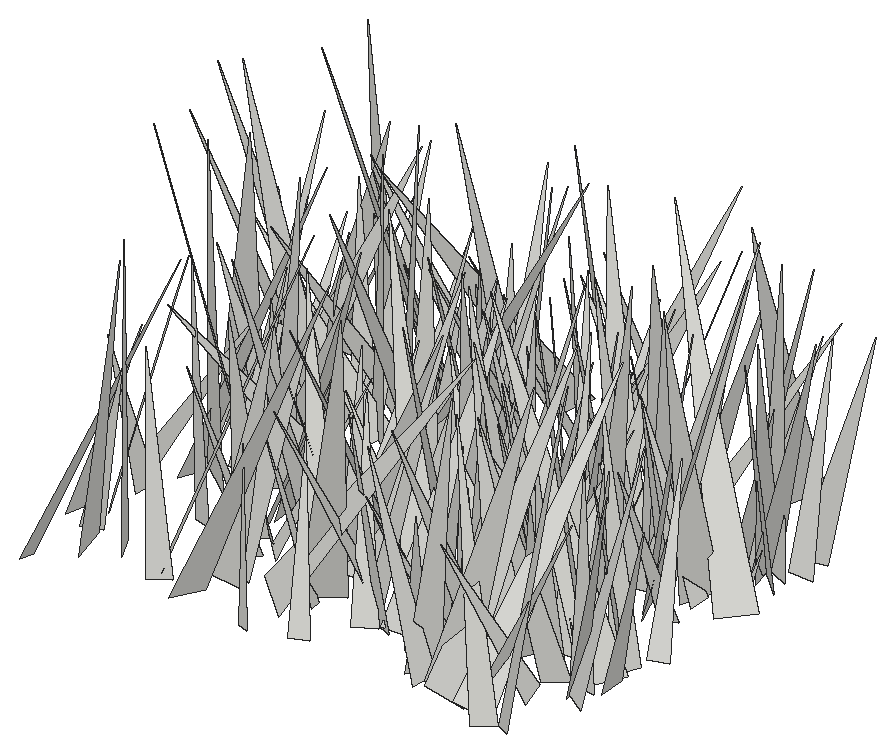
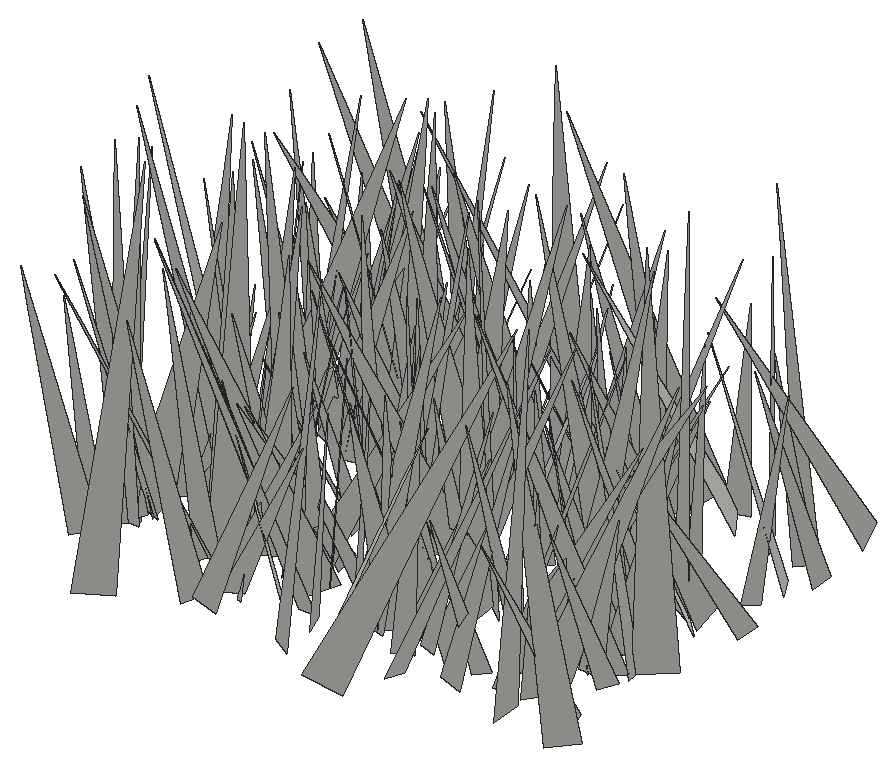
# SketchUp Ruby script. Lengths in inches.
U = 1.inch
M = Sketchup.active_model
def pt(a) = Geom::Point3d.new(a.map { |v| v * U })
def face(e, loops, mat)
  f = e.add_face(loops[0].map { |a| pt(a) })
  loops[1..].each { |l| e.add_face(l.map { |a| pt(a) }).erase! }
  f.material = f.back_material = mat if mat
  f
end
# faces: each face lists its corners as indices into pts; further lists are holes
def faces(e, pts, list, mat = nil) = list.each { |f| face(e, (f[0].is_a?(Array) ? f : [f]).map { |l| l.map { |i| pts[i] } }, mat) }
# xy, xz, yz: faces in a plane at the given z, y or x. An outline is a flat list of corners, or four numbers for a rectangle; further outlines are holes
def ring(l) = l.size == 4 ? [[l[0], l[1]], [l[2], l[1]], [l[2], l[3]], [l[0], l[3]]] : l.each_slice(2).to_a
def flat(e, list, mat, &to3) = list.each { |f| face(e, (f[0].is_a?(Array) ? f : [f]).map { |l| ring(l).map { |u, v| to3.(u, v) } }, mat) }
def xy(e, z, list, mat = nil) = flat(e, list, mat) { |x, y| [x, y, z] }
def xz(e, y, list, mat = nil) = flat(e, list, mat) { |x, z| [x, y, z] }
def yz(e, x, list, mat = nil) = flat(e, list, mat) { |y, z| [x, y, z] }
def lines(e, pts, list) = list.each { |a, b| e.add_line(pt(pts[a]), pt(pts[b])) }
# prism: a flat outline (further loops are holes) pulled along v
def prism(e, loops, v, mat = nil)
  f = face(e, loops, mat); d = Geom::Vector3d.new(v.map { |x| x * U })
  f.pushpull(f.normal.samedirection?(d) ? d.length : -d.length)
end
def box(e, o, s, mat = nil) = prism(e, [[o, [o[0] + s[0], o[1], o[2]], [o[0] + s[0], o[1] + s[1], o[2]], [o[0], o[1] + s[1], o[2]]]], [0, 0, s[2]], mat)
def at(x, y, z, deg = 0) = Geom::Transformation.translation(pt([x, y, z])) * Geom::Transformation.rotation(ORIGIN, Z_AXIS, deg.degrees)
def axes(o, x, y, z) = Geom::Transformation.new([*x, 0, *y, 0, *z, 0, *pt(o).to_a, 1])
def part(name) = M.definitions.add(name)
# library, detail: a bought-in or finely detailed component or shape, given as its bounding box
def library(name, o, s) = part(name).tap { |d| box(d.entities, o, s) }
def detail(e, o, s) = box(e.add_group.entities, o, s)
def put(e, d, t, mat = nil) = e.add_instance(d, t).tap { |i| i.material = mat if mat }
def group(e, t, mat = nil) = e.add_group.tap { |g| g.transformation = t; g.material = mat if mat }.entities
root = M.entities
c1 = part("fur_instance\#9")
p = [[0.8125,0,1.79],[0.67,-0.02,1.48],[0,-0.11,0],[0,0.11,0]]
faces(c1.entities,p,[[0,1,2,3]])
put(root,c1,axes([138.46,445.25,-27.1],[-0.67807,6.71445,3.30984],[6.96597,-0.65101,2.74773],[-2.74118,-3.31527,6.16389]))
put(root,c1,axes([137.26,444.68,-27.1],[-1.4583,4.1794,0.64732],[4.14586,1.27741,1.09233],[-0.83566,-0.95598,4.28962]))
put(root,c1,axes([135.875,436.88,-27.1],[-3.46561,0.71078,2.1355],[1.4755,3.67824,1.17025],[1.69955,-1.74395,3.33859]))
put(root,c1,axes([134.85,433.95,-27.1],[4.46137,-0.22154,0.62784],[-0.29219,-4.4737,0.49769],[-0.59824,0.53291,4.43905]))
put(root,c1,axes([134.64,438.63,-27.1],[3.53802,-1.77872,0.68161],[-1.86523,-2.94336,2.00089],[0.38644,2.07817,3.41729]))
put(root,c1,axes([136.17,445.02,-27.1],[-2.24412,3.20659,0.81725],[3.00578,2.38826,-1.11699],[1.38398,0.01256,3.75108]))
put(root,c1,axes([135.39,447.88,-27.1],[4.11341,0.99659,0.14821],[0.94897,-4.04143,0.83763],[-0.33855,0.78037,4.1487]))
put(root,c1,axes([135.64,435.11,-27.1],[4.69542,3.0157,0.91715],[3.05189,-4.76105,0.03053],[-0.78841,-0.46959,5.58037]))
put(root,c1,axes([137.41,442.85,-27.1],[2.70621,-3.86796,1.26709],[-3.69816,-2.97221,-1.17466],[-1.70008,0.30833,4.57219]))
put(root,c1,axes([134.6875,449.55,-27.1],[2.49015,-6.48815,0.76577],[-6.33726,-2.19962,1.97082],[1.58797,1.39602,6.66429]))
put(root,c1,axes([135.39,443.14,-27.1],[5.72891,-5.77899,0.7373],[-5.79412,-5.75966,-0.12335],[-0.60698,0.43635,8.13646]))
put(root,c1,axes([135.65,430.11,-27.1],[6.20269,2.14266,0.41588],[1.88774,-5.89525,2.21806],[-1.09562,1.97291,6.17613]))
put(root,c1,axes([136.48,439.63,-27.1],[3.1839,3.43631,0.24845],[3.39454,-3.18669,0.57383],[-0.5891,0.20968,4.64932]))
put(root,c1,axes([136.17,433.32,-27.1],[2.52401,-3.24586,0.70539],[-3.32076,-2.44552,0.62916],[0.07602,0.94215,4.0633]))
put(root,c1,axes([141.53,442.02,-27.1],[-3.36679,-6.63148,1.92496],[-6.20382,1.96447,-4.08298],[-3.03226,3.34389,6.21619]))
put(root,c1,axes([137.76,447.41,-27.1],[3.42061,-2.16163,2.16053],[-2.46149,-3.8706,0.02453],[-1.81151,1.17767,4.04631]))
put(root,c1,axes([135.87,443.82,-27.1],[5.69454,1.71793,1.14191],[1.95584,-5.5622,-1.38552],[-0.6557,-1.67144,5.78441]))
put(root,c1,axes([137.82,440.1,-27.1],[1.84381,6.83005,0.32521],[6.75707,-1.87158,0.99709],[-1.04756,-0.05069,7.00393]))
put(root,c1,axes([139.02,443.38,-27.1],[-7.80525,1.8691,2.4402],[2.24771,8.01322,1.05174],[2.09664,-1.63243,7.95672]))
put(root,c1,axes([137.82,449,-27.1],[-7.27615,-1.41209,3.18772],[-1.2687,7.94356,0.62294],[3.24745,-0.06052,7.38568]))
put(root,c1,axes([138.12,432.84,-27.1],[5.01686,3.02729,2.73746],[3.17963,-5.61852,0.38618],[-2.55892,-1.04628,5.84673]))
put(root,c1,axes([137.42,439.07,-27.1],[-3.84702,-6.56229,2.86732],[-6.71624,4.43571,1.14075],[2.48541,1.82909,7.52076]))
put(root,c1,axes([136.5,438.68,-27.1],[6.82155,0.82248,0.97272],[0.53436,-6.65794,1.88216],[-1.15634,1.77527,6.60814]))
put(root,c1,axes([140.33,445.28,-27.1],[-4.08347,2.98679,1.40676],[3.27171,3.36098,2.36101],[-0.44252,-2.71247,4.47451]))
put(root,c1,axes([136.89,432.24,-27.1],[6.91292,1.02767,1.79019],[1.3308,-7.00178,-1.11957],[-1.57792,-1.40299,6.89863]))
put(root,c1,axes([139.17,436.13,-27.1],[1.89742,4.59885,2.05217],[4.78177,-2.33318,0.8074],[-1.57969,-1.53878,4.90894]))
put(root,c1,axes([137.47,444.66,-27.1],[3.73633,3.15118,1.53756],[3.50493,-3.41917,-1.50964],[-0.09758,-2.15258,4.64878]))
put(root,c1,axes([142.22,436.53,-27.1],[-6.33694,-5.31771,1.42218],[-5.44687,5.74429,-2.79146],[-0.79519,3.03026,7.78734]))
put(root,c1,axes([140.46,442.15,-27.1],[-5.57045,-1.42182,0.3414],[-1.0257,4.7578,3.07884],[1.04215,-2.91715,4.85512]))
put(root,c1,axes([139.31,447.74,-27.1],[-5.60645,-3.595,0.79099],[-2.74257,5.04084,3.47133],[2.4552,-2.57833,5.68385]))
put(root,c1,axes([138.93,441.08,-27.1],[6.1687,-0.67373,2.21616],[-0.70194,-6.55164,-0.0379],[-2.20738,0.2006,6.20527]))
put(root,c1,axes([139,446.24,-27.1],[0.94432,5.62245,1.27282],[5.76049,-0.87093,-0.42662],[0.22085,-1.32412,5.68522]))
put(root,c1,axes([136.49,444.21,-27.1],[1.93796,6.92662,2.2466],[6.80944,-0.90011,-3.09877],[2.58009,-2.82714,6.49087]))
put(root,c1,axes([142.74,446.75,-27.1],[-5.1387,-6.17044,1.38685],[-6.22365,4.61615,-2.52214],[-1.12419,2.64967,7.62361]))
put(root,c1,axes([137.97,442.4,-27.1],[3.87779,-2.1954,0.31482],[-2.2129,-3.78759,0.8446],[0.14815,0.88911,4.37535]))
put(root,c1,axes([140.57,431.82,-27.1],[1.59272,-3.9303,2.28796],[-4.37909,-1.9795,-0.352],[-1.22702,1.96293,4.22612]))
put(root,c1,axes([140.82,448.55,-27.1],[-1.81224,-5.34948,0.90018],[-5.42401,1.80193,-0.21131],[0.08596,0.92064,5.64415]))
put(root,c1,axes([139.6,437.65,-27.1],[2.64561,4.33348,1.24236],[4.47199,-2.70465,-0.08904],[-0.56902,-1.10798,5.07645]))
put(root,c1,axes([139.79,439.99,-27.1],[3.06125,-3.87557,0.82155],[-3.90702,-3.12527,-0.1848],[-0.65588,0.52812,4.93529]))
put(root,c1,axes([142.3,435.47,-27.1],[-1.49858,-3.44059,1.04989],[-3.40031,0.98374,-1.62968],[-1.17382,1.54281,3.38047]))
put(root,c1,axes([140.17,445.26,-27.1],[-3.26006,-5.04679,2.60885],[-5.29814,3.78652,0.70434],[2.05082,1.75965,5.96674]))
put(root,c1,axes([140.4,447.2,-27.1],[-1.29453,3.3269,0.92168],[3.25121,1.50588,-0.8692],[1.16077,-0.50757,3.46245]))
put(root,c1,axes([142.85,449.34,-27.1],[-6.28485,-0.79991,0.77187],[-0.56549,6.11624,1.73401],[0.95701,-1.63912,6.09364]))
put(root,c1,axes([140.27,432.24,-27.1],[5.9455,4.2001,0.21568],[4.05072,-5.81939,1.66213],[-1.13095,1.23699,7.08711]))
put(root,c1,axes([141.33,436.36,-27.1],[3.50702,-4.68842,0.88051],[-4.69288,-3.58696,-0.4079],[-0.85643,0.45629,5.84073]))
put(root,c1,axes([141.22,437.29,-27.1],[3.86213,1.08614,0.2172],[1.09096,-3.86634,-0.0646],[-0.19154,-0.12107,4.01143]))
put(root,c1,axes([143.96,437.25,-27.1],[-0.89834,-6.55906,1.37521],[-6.65422,0.70817,-0.96916],[-0.7961,1.48213,6.54897]))
put(root,c1,axes([143.14,447.02,-27.1],[-1.82356,-4.42835,0.39133],[-4.41286,1.85435,0.42054],[0.53859,0.19978,4.77062]))
put(root,c1,axes([144.49,451.57,-27.1],[4.16443,-6.48584,0.7003],[-5.50995,-3.94185,-3.74183],[-3.49241,-1.51483,6.7385]))
put(root,c1,axes([144.28,446.5,-27.1],[-0.56318,-3.80765,0.20803],[-3.75255,0.51599,-0.71463],[-0.67806,0.30692,3.78215]))
put(root,c1,axes([141.12,438.875,-27.1],[7.51831,-0.309,0.51299],[-0.23256,-7.46002,-1.08516],[-0.55186,-1.06592,7.446]))
put(root,c1,axes([143.74,439.35,-27.1],[-2.47,2.58512,1.49197],[2.74392,2.72878,-0.18549],[1.17462,-0.93843,3.57063]))
put(root,c1,axes([143,443.21,-27.1],[-4.52397,-6.09316,3.51067],[-6.34353,5.33763,1.08955],[3.03497,2.07386,7.51038]))
put(root,c1,axes([144.87,440.02,-27.1],[-3.28468,-3.33783,0.1825],[-3.30088,3.27904,0.56182],[0.52783,-0.26523,4.64915]))
put(root,c1,axes([142.43,433.98,-27.1],[0.67083,5.9533,2.27987],[6.17356,-0.03505,-1.72498],[1.58958,-2.37626,5.73727]))
put(root,c1,axes([142.48,433.25,-27.1],[1.87666,-6.19619,1.68038],[-6.32701,-1.4881,1.57887],[1.08876,2.03251,6.27868]))
put(root,c1,axes([142.64,436.03,-27.1],[3.00056,3.161,0.00616],[3.13284,-2.97269,-0.58633],[0.42105,-0.40809,4.31874]))
put(root,c1,axes([144.56,443.53,-27.1],[-0.28609,-7.90952,0.17476],[-7.91116,0.28452,-0.07401],[-0.06767,0.17732,7.91434]))
put(root,c1,axes([144.39,438.13,-27.1],[-3.15103,-4.03715,0.66571],[-3.75697,3.18756,1.54769],[1.62077,-0.46003,4.88182]))
put(root,c1,axes([146.35,433.85,-27.1],[-3.92472,-1.58946,0.29836],[-1.61245,3.78584,-1.04222],[-0.12416,1.07696,4.10409]))
put(root,c1,axes([143.62,447.89,-27.1],[0.2783,-5.0487,0.14304],[-4.93686,-0.24166,1.07529],[1.0664,0.19877,4.94071]))
put(root,c1,axes([144.15,443.14,-27.1],[3.92282,-1.4058,1.44453],[-1.66907,-4.03753,0.60333],[-1.1301,1.0833,4.1232]))
put(root,c1,axes([146.07,447.01,-27.1],[-0.62718,-6.98929,2.39617],[-7.29856,0.2117,-1.29283],[-1.15016,2.46782,6.89725]))
put(root,c1,axes([145.92,434.93,-27.1],[2.97491,-4.25566,3.74848],[-5.0806,-3.88069,-0.37363],[-2.51977,2.80026,5.17891]))
put(root,c1,axes([145.31,430.88,-27.1],[1.49909,3.09185,1.25062],[3.12666,-1.78006,0.6529],[-1.16087,-0.8017,3.3735]))
put(root,c1,axes([145.91,449.82,-27.1],[-3.80651,-3.12707,0.03174],[-3.06593,3.74155,0.93273],[0.61617,-0.70095,4.83716]))
put(root,c1,axes([142.07,431.61,-27.1],[7.97011,-1.5942,0.50435],[-1.65185,-7.88792,1.1707],[-0.25934,1.24806,8.04323]))
put(root,c1,axes([145.84,445.64,-27.1],[-5.09281,3.29268,0.78292],[3.01884,5.05892,-1.63872],[1.53013,0.9783,5.83893]))
put(root,c1,axes([144.82,442.04,-27.1],[-1.49682,6.02983,3.22428],[6.74332,1.8484,-0.32627],[1.1325,-3.03643,6.20426]))
put(root,c1,axes([145.1,446.67,-27.1],[-2.61332,3.50076,2.27341],[3.90248,3.00092,-0.13507],[1.48133,-1.72983,4.36652]))
put(root,c1,axes([145.95,443.05,-27.1],[0.78964,4.34465,0.57519],[4.335,-0.86018,0.54605],[-0.64386,-0.46311,4.38193]))
put(root,c1,axes([146.01,441.5,-27.1],[2.63979,2.66437,0.28601],[2.37928,-2.51517,1.47039],[-1.23275,0.85099,3.4504]))
put(root,c1,axes([147.05,445.27,-27.1],[0.66208,3.60921,1.19442],[3.54519,-1.02396,1.12897],[-1.37285,-0.90361,3.49144]))
put(root,c1,axes([145.29,446.49,-27.1],[4.67947,-2.49587,0.44393],[-2.29207,-4.56374,-1.49753],[-1.08298,-1.12554,5.08765]))
put(root,c1,axes([143.25,443.24,-27.1],[7.82793,-0.68601,0.13891],[-0.69946,-7.6099,1.83483],[0.02566,1.8399,7.64072]))
put(root,c1,axes([145.86,436.43,-27.1],[-1.59343,4.55905,1.08338],[4.45907,1.82697,-1.12985],[1.44061,-0.61229,4.69546]))
put(root,c1,axes([145.58,444.2,-27.1],[5.69502,0.05498,1.49404],[0.36012,-5.7612,-1.16071],[-1.45103,-1.21405,5.57575]))
put(root,c1,axes([147.49,441.54,-27.1],[-3.18847,2.06393,0.29466],[1.98964,3.17316,-0.69666],[0.62286,0.42918,3.73374]))
put(root,c1,axes([146.5,442.32,-27.1],[4.01654,5.38759,0.39242],[5.219,-3.99648,1.45013],[-1.3936,0.56102,6.56169]))
put(root,c1,axes([148.5,437.5,-27.1],[-3.99734,1.08155,0.32432],[1.12476,3.91891,0.79421],[0.09918,-0.85212,4.0642]))
put(root,c1,axes([147.4375,431.52,-27.1],[-1.47,3.64091,0.87512],[3.73843,1.4809,0.11844],[0.21496,-0.85654,3.92467]))
put(root,c1,axes([147.6,448.16,-27.1],[-4.30965,-1.39305,1.63599],[-1.58025,4.5392,-0.29767],[1.45598,0.80324,4.51941]))
put(root,c1,axes([146.3125,445.99,-27.1],[-4.08433,-4.26667,3.28401],[-4.58243,4.91876,0.69141],[2.82675,1.80893,5.86585]))
put(root,c1,axes([149.05,437.01,-27.1],[2.27452,-5.56414,4.58515],[-6.58849,-3.55674,-1.04785],[-2.92831,3.68058,5.91904]))
put(root,c1,axes([147.09,443.36,-27.1],[-3.51133,-6.12863,1.17286],[-5.90116,3.69891,1.66117],[2.0278,0.152,6.86513]))
put(root,c1,axes([148.38,437.23,-27.1],[-2.55623,-6.61752,0.06611],[-6.61278,2.55692,0.25211],[0.25899,-0.02922,7.08959]))
put(root,c1,axes([147.51,450.23,-27.1],[-4.05006,-5.82532,2.03849],[-5.82326,4.4146,1.04584],[2.04438,1.03428,7.01738]))
put(root,c1,axes([148.43,435.33,-27.1],[-4.62318,-3.47557,0.41553],[-3.19467,4.47097,1.85217],[1.4305,-1.24775,5.47931]))
put(root,c1,axes([147.75,445.39,-27.1],[-1.86728,-3.21645,1.13397],[-3.16749,2.11482,0.78275],[1.26429,0.54787,3.63587]))
put(root,c1,axes([146.36,436.55,-27.1],[0.74046,6.81709,2.01452],[6.9144,-0.22063,-1.79488],[1.64984,-2.13492,6.61811]))
put(root,c1,axes([150.45,444.42,-27.1],[-1.24481,-6.10899,0.55091],[-5.80958,0.99391,-2.10566],[-1.96776,0.93016,5.86818]))
put(root,c1,axes([146.16,434.57,-27.1],[5.23004,-6.31048,0.45418],[-6.32662,-5.22094,0.31214],[-0.04891,0.54893,8.19012]))
put(root,c1,axes([148.82,433.72,-27.1],[-2.21571,3.96483,0.99922],[4.07213,2.24229,0.13245],[0.36886,-0.93805,4.54001]))
put(root,c1,axes([145.53,436.58,-27.1],[5.33015,-4.46349,0.382],[-4.4244,-5.15196,1.5366],[0.7024,1.41905,6.78027]))
put(root,c1,axes([148.25,434.95,-27.1],[3.95249,6.61953,0.92655],[6.54498,-4.05132,1.02412],[-1.35642,-0.25967,7.64143]))
put(root,c1,axes([149.41,434.05,-27.1],[1.51862,3.68557,2.40948],[4.21899,-1.94756,0.31991],[-1.2606,-2.07817,3.97332]))
put(root,c1,axes([149.16,445.26,-27.1],[-3.54566,-2.66431,1.6705],[-2.78653,3.82874,0.19209],[1.45754,0.83849,4.43096]))
put(root,c1,axes([149.42,439.99,-27.1],[-4.67336,-1.61213,2.14084],[-2.03116,4.93814,-0.71533],[1.7483,1.42769,4.89159]))
put(root,c1,axes([147.56,438.25,-27.1],[3.87683,-5.48097,2.21285],[-5.90731,-3.50163,1.67625],[0.20355,2.76859,6.50085]))
put(root,c1,axes([144.63,433.45,-27.1],[4.68753,6.76488,0.69054],[6.04009,-3.75687,-4.19721],[3.12373,-2.88717,7.07954]))
put(root,c1,axes([151.45,448.19,-27.1],[-3.62089,2.64212,0.01483],[2.58278,3.53416,0.96476],[-0.55698,-0.78788,4.37731]))
put(root,c1,axes([150.62,444.22,-27.1],[-4.55116,2.07867,0.64916],[1.93391,4.54938,-1.00919],[1.00113,0.66152,4.90056]))
put(root,c1,axes([148.16,444.66,-27.1],[1.07989,-3.22676,1.49499],[-3.22529,-0.23045,1.83235],[1.49815,1.82977,2.86716]))
put(root,c1,axes([152,447.87,-27.1],[-4.37284,2.10544,0.41102],[2.13916,4.20984,1.19366],[-0.16073,-1.25217,4.70423]))
put(root,c1,axes([151.1,445.63,-27.1],[-4.28874,-2.62611,1.19653],[-2.76089,4.3576,-0.33198],[0.84,0.91449,5.01792]))
put(root,c1,axes([149.01,441.76,-27.1],[-2.72966,-3.54913,3.67888],[-4.47058,3.67982,0.23296],[2.47878,2.72838,4.47136]))
put(root,c1,axes([151.71,449.55,-27.1],[-0.61117,-4.98438,1.28841],[-4.9544,0.21679,-1.51148],[-1.3993,1.40945,4.78884]))
put(root,c1,axes([152.01,437.91,-27.1],[-4.80614,1.67739,0.07303],[1.63862,4.73444,-0.90443],[0.36591,0.83033,5.00945]))
put(root,c1,axes([152.04,436.93,-27.1],[-4.34264,3.05124,0.46122],[3.07623,4.34339,0.23041],[0.24406,-0.45414,5.3024]))
put(root,c1,axes([148.8,448.32,-27.1],[3.81482,2.67004,0.71919],[2.75746,-3.58156,-1.32965],[0.20681,-1.49748,4.4625]))
put(root,c1,axes([149.95,438.84,-27.1],[-0.40221,-7.56998,1.93164],[-7.73436,0.65878,0.97125],[1.10251,1.85984,7.51818]))
put(root,c1,axes([149.92,437.72,-27.1],[-3.16207,-7.07316,1.24758],[-6.76016,3.39142,2.09364],[2.42619,0.2311,7.45956]))
put(root,c1,axes([149.51,443.8,-27.1],[3.96425,-0.56902,0.64503],[-0.79665,-3.57598,1.74151],[-0.32433,1.82859,3.60641]))
put(root,c1,axes([151.75,435.0625,-27.1],[-3.32799,-2.15223,0.18164],[-2.02775,3.22824,1.09879],[0.74386,-0.82886,3.80792]))
put(root,c1,axes([150.16,434.19,-27.1],[-2.57926,6.41675,1.59968],[6.21683,2.93816,-1.76197],[2.25493,-0.76079,6.68751]))
put(root,c1,axes([152.11,445.125,-27.1],[-4.3858,5.26104,2.02142],[5.54364,4.48874,0.34523],[1.01623,-1.78118,6.84066]))
put(root,c1,axes([150.25,441.11,-27.1],[0.10364,-5.95888,1.80759],[-6.13378,0.21397,1.05707],[1.07352,1.79787,5.86529]))
put(root,c1,axes([150.87,441.42,-27.1],[4.041,0.55824,1.1889],[0.26805,-4.11576,1.02147],[-1.28579,0.89645,3.94942]))
put(root,c1,axes([151.73,443.16,-27.1],[-3.94545,3.07895,0.18102],[2.74281,3.63702,-2.08047],[1.41057,1.53994,4.55172]))
put(root,c1,axes([148.375,447.62,-27.1],[4.07945,6.65627,1.20942],[6.56454,-3.55321,-2.58689],[1.63565,-2.3408,7.36585]))
put(root,c1,axes([151.07,445.1,-27.1],[3.64038,-1.44849,0.64201],[-1.22649,-3.59476,-1.15586],[-1.003,-0.8615,3.74359]))
put(root,c1,axes([150.91,448.48,-27.1],[-2.708,-3.38854,1.07596],[-2.8715,2.88211,1.84961],[2.09627,-0.42942,3.92357]))
put(root,c1,axes([150.86,435.49,-27.1],[4.29298,-1.68508,0.76366],[-1.68331,-4.35833,-0.1541],[-0.76754,0.13347,4.60928]))
put(root,c1,axes([151.11,443.92,-27.1],[4.61454,1.12705,1.27743],[1.23829,-4.75228,-0.2803],[-1.16993,-0.58453,4.7419]))
put(root,c1,axes([148.93,445.96,-27.1],[3.61026,-5.57217,1.81458],[-5.57053,-2.60139,3.09478],[1.81959,3.09184,5.87413]))
put(root,c1,axes([153.03,431.99,-27.1],[-4.85785,0.78834,1.37895],[1.02249,4.94749,0.77364],[1.21552,-1.0112,4.86021]))
put(root,c1,axes([150.88,438.12,-27.1],[2.46673,-5.38252,0.46134],[-5.39282,-2.42347,0.55987],[0.31917,0.65147,5.89431]))
put(root,c1,axes([151.18,436.8,-27.1],[4.40781,-2.35415,1.32075],[-2.57038,-4.43283,0.67704],[-0.82436,1.23418,4.95101]))
put(root,c1,axes([152.36,435.94,-27.1],[-5.45284,-1.57742,1.94379],[-0.6971,5.43147,2.45217],[2.40429,-2.00271,5.11943]))
put(root,c1,axes([151.23,437.03,-27.1],[4.54007,-1.04122,1.07478],[-1.33062,-4.37982,1.37772],[-0.68465,1.60765,4.44952]))
put(root,c1,axes([151.49,433.46,-27.1],[1.84889,-3.8875,0.07331],[-3.87281,-1.83403,0.41727],[0.34554,0.24513,4.2845]))
put(root,c1,axes([151.92,444.05,-27.1],[-1.54169,4.36128,2.00643],[4.43238,2.10262,-1.16464],[1.84406,-1.40768,4.47674]))
put(root,c1,axes([151.81,440.87,-27.1],[1.90499,3.12749,0.05078],[3.06447,-1.8542,-0.76405],[0.62675,-0.43991,3.5814]))
put(root,c1,axes([153.87,436.09,-27.1],[-5.4764,4.5647,2.90915],[5.14181,5.68019,0.76664],[1.69155,-2.48788,7.08799]))
put(root,c1,axes([155.55,437.24,-27.1],[-0.37721,6.24874,2.25952],[6.16262,-0.51732,2.45945],[-2.4848,-2.23161,5.75674]))
put(root,c1,axes([152.54,432.53,-27.1],[5.43979,-3.16023,1.66658],[-3.30816,-5.60189,0.17546],[-1.34931,0.9938,6.28869]))
put(root,c1,axes([154.05,437.64,-27.1],[2.81422,-5.9892,1.8303],[-5.99838,-3.15452,-1.09945],[-1.79999,1.14839,6.52546]))
put(root,c1,axes([154.875,437,-27.1],[-4.89111,-2.11302,1.38613],[-2.21595,5.03778,-0.13961],[1.21481,0.68196,5.3262]))
put(root,c1,axes([154.67,442.26,-27.1],[-0.07394,-6.12578,2.47714],[-6.56947,-0.19789,-0.68546],[-0.70961,2.47033,6.08776]))
put(root,c1,axes([152.29,449.41,-27.1],[5.3173,-1.56529,0.48292],[-1.59322,-5.32309,0.28875],[-0.38078,0.41424,5.53538]))
put(root,c1,axes([154.28,432.92,-27.1],[-2.72992,2.63061,1.69887],[2.87463,2.99911,-0.02472],[1.24209,-1.1593,3.79104]))
put(root,c1,axes([152.375,444.22,-27.1],[6.025,3.41302,0.55167],[3.40656,-6.04972,0.22351],[-0.59027,-0.07668,6.92094]))
put(root,c1,axes([155.33,436.25,-27.1],[-1.95958,-4.83915,1.26512],[-4.97855,2.01787,0.00704],[0.48156,1.1699,5.22085]))
put(root,c1,axes([155.62,439.08,-27.1],[-2.21382,-3.77344,0.32599],[-3.76288,2.23425,0.30817],[0.43109,0.1241,4.36404]))
put(root,c1,axes([153.91,441.43,-27.1],[6.97924,-1.80721,1.76653],[-1.77915,-7.19853,-0.33521],[-1.79479,0.10824,7.20163]))
put(root,c1,axes([156.9,430.67,-27.1],[-0.83276,5.81039,0.96307],[5.68734,0.54058,1.65638],[-1.53047,-1.15272,5.63121]))
put(root,c1,axes([153.75,445.42,-27.1],[4.25947,-6.86655,0.67935],[-6.89421,-4.26807,0.08653],[-0.2843,0.62304,8.07992]))
put(root,c1,axes([155.875,436.74,-27.1],[0.35449,6.1752,1.09899],[6.2119,-0.49795,0.79425],[-0.86782,-1.04187,6.13416]))
put(root,c1,axes([154.02,445.33,-27.1],[3.44417,-6.15496,0.43731],[-6.17002,-3.42915,0.33004],[0.07525,0.54268,7.04535]))
put(root,c1,axes([153.87,446.68,-27.1],[5.53978,-0.90724,0.62547],[-0.85463,-5.56113,-0.49688],[-0.69563,-0.39269,5.59154]))
put(root,c1,axes([158.34,436.06,-27.1],[-5.06971,5.94983,1.91077],[6.22333,4.58369,2.23904],[-0.56711,-2.88838,7.48926]))
put(root,c1,axes([156.03,442.62,-27.1],[-1.67476,-3.89018,1.26522],[-4.03938,1.78862,0.15259],[0.64624,1.09838,4.23261]))
put(root,c1,axes([156.96,434.92,-27.1],[0.96308,-5.75121,1.64983],[-5.7805,-1.32563,-1.24675],[-1.54408,1.37555,5.69645]))
put(root,c1,axes([154.93,436.03,-27.1],[3.91329,-2.80057,0.16354],[-2.76188,-3.89534,-0.61821],[-0.49189,-0.40864,4.7723]))
put(root,c1,axes([155.8,436.07,-27.1],[1.04102,-4.92803,1.21287],[-5.07408,-1.03535,0.14838],[-0.10125,1.21771,5.0346]))
put(root,c1,axes([157.33,442.93,-27.1],[-4.29082,0.07848,0.62907],[0.12494,4.3243,0.31276],[0.62151,-0.32753,4.28013]))
put(root,c1,axes([156.85,433.65,-27.1],[-4.22388,-0.55824,1.0602],[-0.01996,3.91714,1.98304],[1.19803,-1.90295,3.77099]))
put(root,c1,axes([159.06,442.99,-27.1],[-3.56857,7.17935,0.49748],[7.02506,3.35468,1.97986],[-1.56176,-1.31463,7.76903]))
put(root,c1,axes([154,432.15,-27.1],[4.37755,-6.1842,1.75356],[-6.40379,-4.01166,1.83857],[0.55746,2.47882,7.3503]))
put(root,c1,axes([154.4,431.46,-27.1],[-0.17327,7.80384,1.95788],[7.72096,0.71202,-2.15474],[2.26272,-1.83203,7.50246]))
put(root,c1,axes([157.79,435.71,-27.1],[-4.59653,-5.39297,2.39685],[-5.86856,4.49796,-1.13384],[0.62378,2.57709,6.99476]))
put(root,c1,axes([157.86,435.43,-27.1],[-3.7674,-0.4134,0.34529],[-0.49063,3.64055,-0.99453],[0.22227,1.02903,3.6572]))
put(root,c1,axes([155.44,451.49,-27.1],[6.81384,-4.6319,0.82302],[-4.34734,-6.75311,-2.01405],[-1.7979,-1.22528,7.98915]))
put(root,c1,axes([153.79,446.69,-27.1],[3.84668,4.92623,0.09388],[4.62666,-3.57049,-2.21792],[1.69428,-1.43435,5.84342]))
put(root,c1,axes([155.87,431.28,-27.1],[-2.00066,7.03095,0.19663],[6.73059,1.97306,-2.06922],[2.04255,0.38513,7.01108]))
put(root,c1,axes([155.84,441.75,-27.1],[5.68987,2.39384,1.65752],[2.61602,-5.80047,-0.60296],[-1.2784,-1.21517,6.14342]))
put(root,c1,axes([157.32,441.16,-27.1],[0.58704,-3.79537,0.45103],[-3.78334,-0.64184,-0.47675],[-0.5428,0.36891,3.81079]))
put(root,c1,axes([156.51,437.45,-27.1],[4.13906,-0.88394,1.08396],[-0.87234,-4.27812,-0.15771],[-1.09332,0.06702,4.22946]))
put(root,c1,axes([157.63,430.9,-27.1],[3.93388,5.26717,1.14139],[4.90502,-4.08461,1.94372],[-2.23307,0.30691,6.28017]))
put(root,c1,axes([155.79,431.69,-27.1],[4.34496,-0.35551,0.43941],[-0.4633,-4.19131,1.19014],[-0.32376,1.22666,4.19388]))
put(root,c1,axes([155.06,443.27,-27.1],[-0.81294,-7.33898,4.00432],[-7.82592,2.08335,2.22952],[2.94113,3.51498,7.03923]))
put(root,c1,axes([157.11,443.28,-27.1],[6.05759,-4.04132,1.47541],[-3.82561,-6.22554,-1.34569],[-1.96821,-0.33746,7.15653]))
put(root,c1,axes([158.46,437.16,-27.1],[-4.8782,2.33838,1.88669],[2.5546,5.12175,0.25721],[1.58166,-1.06025,5.40358]))
put(root,c1,axes([157.97,435.15,-27.1],[0.13174,-4.85064,1.64659],[-5.10405,0.01535,0.4536],[0.43432,1.65178,4.83118]))
put(root,c1,axes([156.08,441.52,-27.1],[7.78659,2.72532,1.24866],[2.87625,-7.77148,-0.97412],[-0.84485,-1.33952,8.19204]))
put(root,c1,axes([157.5,444.74,-27.1],[6.67173,1.075,1.66778],[0.88806,-6.84957,0.86244],[-1.77439,0.61387,6.70252]))
put(root,c1,axes([158.93,438.49,-27.1],[-1.59242,3.59476,0.56652],[3.61736,1.63113,-0.18207],[0.39739,-0.44291,3.92746]))
put(root,c1,axes([158.16,437.44,-27.1],[-3.52584,-3.38703,1.52089],[-2.9555,3.82986,1.67745],[2.24724,-0.27722,4.59235]))
put(root,c1,axes([157.51,445.4,-27.1],[2.91311,4.64162,1.0633],[4.76072,-2.81168,-0.76908],[0.10392,-1.30816,5.4258]))
put(root,c1,axes([157.94,446.45,-27.1],[-1.4348,-7.0433,2.45033],[-7.23254,1.92235,1.29061],[1.81726,2.08982,7.07114]))
put(root,c1,axes([159.04,446.83,-27.1],[-0.27729,4.76979,1.49646],[4.98187,0.38774,-0.31274],[0.41383,-1.47171,4.7676]))
put(root,c1,axes([158.41,434.2,-27.1],[2.85218,4.71528,1.10181],[4.83661,-2.83604,-0.38317],[-0.23454,-1.14272,5.49745]))
put(root,c1,axes([157.8,446.46,-27.1],[7.1612,-0.61813,1.17268],[-0.1707,-6.81898,-2.55193],[-1.31459,-2.48182,6.71956]))
put(root,c1,axes([158.18,445.97,-27.1],[-3.37811,-5.89928,1.5704],[-5.1932,3.72048,2.80499],[3.2091,-0.18922,6.19235]))
put(root,c1,axes([157.73,435.13,-27.1],[5.98567,0.36805,0.66862],[0.55714,-5.71998,-1.83907],[-0.52163,-1.88604,5.70802]))
put(root,c1,axes([157.85,446.15,-27.1],[6.64533,-1.36705,0.39109],[-1.31179,-6.61549,-0.83466],[-0.54862,-0.74069,6.73295]))
put(root,c1,axes([158.65,447.99,-27.1],[3.34726,-4.07819,1.53745],[-4.35777,-3.09938,1.26621],[0.07255,1.99042,5.12177]))
put(root,c1,axes([158.81,435.91,-27.1],[4.67229,-0.63233,0.28263],[-0.57173,-4.60903,-0.86025],[-0.39095,-0.81674,4.63574]))
